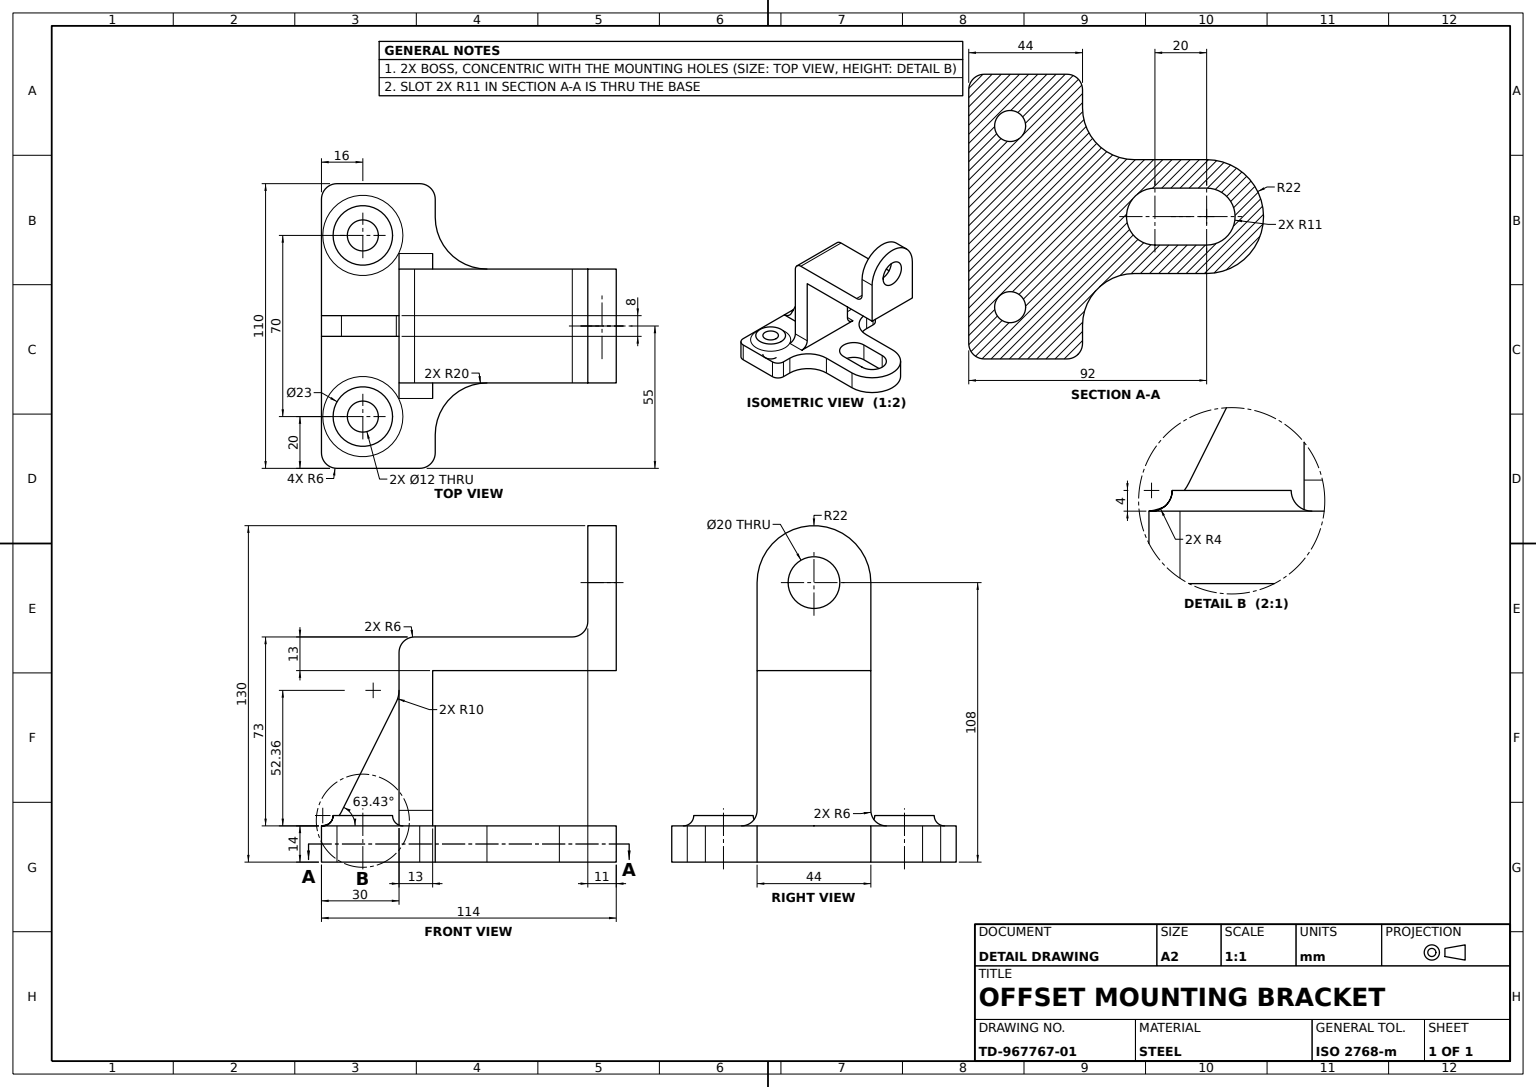
ISO-10303-21;
HEADER;
FILE_DESCRIPTION((''),'2;1');
FILE_NAME('','',(''),(''),'','','');
FILE_SCHEMA(('AUTOMOTIVE_DESIGN'));
ENDSEC;
DATA;
#1=APPLICATION_CONTEXT('');
#2=PRODUCT_CONTEXT('',#1,'mechanical');
#3=PRODUCT('','','',(#2));
#4=PRODUCT_DEFINITION_FORMATION('','',#3);
#5=PRODUCT_DEFINITION_CONTEXT('',#1,'design');
#6=PRODUCT_DEFINITION('','',#4,#5);
#7=PRODUCT_DEFINITION_SHAPE('','',#6);
#8=(LENGTH_UNIT()NAMED_UNIT(*)SI_UNIT(.MILLI.,.METRE.));
#9=(NAMED_UNIT(*)PLANE_ANGLE_UNIT()SI_UNIT($,.RADIAN.));
#10=(NAMED_UNIT(*)SI_UNIT($,.STERADIAN.)SOLID_ANGLE_UNIT());
#11=UNCERTAINTY_MEASURE_WITH_UNIT(LENGTH_MEASURE(1.E-05),#8,'distance_accuracy_value','');
#12=(GEOMETRIC_REPRESENTATION_CONTEXT(3)GLOBAL_UNCERTAINTY_ASSIGNED_CONTEXT((#11))GLOBAL_UNIT_ASSIGNED_CONTEXT((#8,#9,#10))REPRESENTATION_CONTEXT('',''));
#13=CARTESIAN_POINT('',(22.,20.,-43.));
#14=VERTEX_POINT('',#13);
#15=CARTESIAN_POINT('',(28.,14.,-43.));
#16=VERTEX_POINT('',#15);
#17=CARTESIAN_POINT('',(28.,20.,-43.));
#18=DIRECTION('',(0.,0.,1.));
#19=DIRECTION('',(0.,-1.,0.));
#20=AXIS2_PLACEMENT_3D('',#17,#18,#19);
#21=CIRCLE('',#20,6.);
#22=EDGE_CURVE('',#14,#16,#21,.T.);
#23=ORIENTED_EDGE('',*,*,#22,.T.);
#24=CARTESIAN_POINT('',(-28.,14.,-43.));
#25=VERTEX_POINT('',#24);
#26=CARTESIAN_POINT('',(22.,14.,-43.));
#27=DIRECTION('',(-1.,0.,0.));
#28=VECTOR('',#27,1000.);
#29=LINE('',#26,#28);
#30=EDGE_CURVE('',#16,#25,#29,.T.);
#31=ORIENTED_EDGE('',*,*,#30,.T.);
#32=CARTESIAN_POINT('',(-22.,20.,-43.));
#33=VERTEX_POINT('',#32);
#34=CARTESIAN_POINT('',(-28.,20.,-43.));
#35=AXIS2_PLACEMENT_3D('',#34,#18,#19);
#36=CIRCLE('',#35,6.);
#37=EDGE_CURVE('',#25,#33,#36,.T.);
#38=ORIENTED_EDGE('',*,*,#37,.T.);
#39=CARTESIAN_POINT('',(-22.,74.,-43.));
#40=VERTEX_POINT('',#39);
#41=DIRECTION('',(0.,1.,0.));
#42=VECTOR('',#41,1000.);
#43=LINE('',#39,#42);
#44=EDGE_CURVE('',#33,#40,#43,.T.);
#45=ORIENTED_EDGE('',*,*,#44,.T.);
#46=CARTESIAN_POINT('',(22.,74.,-43.));
#47=VERTEX_POINT('',#46);
#48=LINE('',#46,#28);
#49=EDGE_CURVE('',#47,#40,#48,.T.);
#50=ORIENTED_EDGE('',*,*,#49,.F.);
#51=LINE('',#46,#42);
#52=EDGE_CURVE('',#14,#47,#51,.T.);
#53=ORIENTED_EDGE('',*,*,#52,.F.);
#54=EDGE_LOOP('',(#23,#31,#38,#45,#50,#53));
#55=FACE_OUTER_BOUND('',#54,.T.);
#56=AXIS2_PLACEMENT_3D('',#46,#18,#19);
#57=PLANE('',#56);
#58=ADVANCED_FACE('',(#55),#57,.F.);
#59=CARTESIAN_POINT('',(-35.,18.,-4.5));
#60=VERTEX_POINT('',#59);
#61=CARTESIAN_POINT('',(-35.,18.,-27.5));
#62=VERTEX_POINT('',#61);
#63=CARTESIAN_POINT('',(-35.,18.,-16.));
#64=AXIS2_PLACEMENT_3D('',#63,#41,#18);
#65=CIRCLE('',#64,11.5);
#66=EDGE_CURVE('',#60,#62,#65,.T.);
#67=ORIENTED_EDGE('',*,*,#66,.T.);
#68=EDGE_CURVE('',#62,#60,#65,.T.);
#69=ORIENTED_EDGE('',*,*,#68,.T.);
#70=EDGE_LOOP('',(#67,#69));
#71=FACE_OUTER_BOUND('',#70,.T.);
#72=CARTESIAN_POINT('',(-35.,18.,-10.));
#73=VERTEX_POINT('',#72);
#74=CARTESIAN_POINT('',(-35.,18.,-22.));
#75=VERTEX_POINT('',#74);
#76=CIRCLE('',#64,6.);
#77=EDGE_CURVE('',#73,#75,#76,.T.);
#78=ORIENTED_EDGE('',*,*,#77,.F.);
#79=EDGE_CURVE('',#75,#73,#76,.T.);
#80=ORIENTED_EDGE('',*,*,#79,.F.);
#81=EDGE_LOOP('',(#78,#80));
#82=FACE_BOUND('',#81,.T.);
#83=PLANE('',#64);
#84=ADVANCED_FACE('',(#71,#82),#83,.T.);
#85=CARTESIAN_POINT('',(-35.,0.,-10.));
#86=VERTEX_POINT('',#85);
#87=CARTESIAN_POINT('',(-35.,0.,-22.));
#88=VERTEX_POINT('',#87);
#89=CARTESIAN_POINT('',(-35.,0.,-16.));
#90=AXIS2_PLACEMENT_3D('',#89,#41,#18);
#91=CIRCLE('',#90,6.);
#92=EDGE_CURVE('',#86,#88,#91,.T.);
#93=ORIENTED_EDGE('',*,*,#92,.F.);
#94=LINE('',#85,#42);
#95=EDGE_CURVE('',#86,#73,#94,.T.);
#96=ORIENTED_EDGE('',*,*,#95,.T.);
#97=ORIENTED_EDGE('',*,*,#77,.T.);
#98=LINE('',#87,#42);
#99=EDGE_CURVE('',#88,#75,#98,.T.);
#100=ORIENTED_EDGE('',*,*,#99,.F.);
#101=EDGE_LOOP('',(#93,#96,#97,#100));
#102=FACE_OUTER_BOUND('',#101,.T.);
#103=CYLINDRICAL_SURFACE('',#90,6.);
#104=ADVANCED_FACE('',(#102),#103,.F.);
#105=CARTESIAN_POINT('',(35.,18.,-27.5));
#106=VERTEX_POINT('',#105);
#107=CARTESIAN_POINT('',(35.,18.,-4.5));
#108=VERTEX_POINT('',#107);
#109=CARTESIAN_POINT('',(35.,18.,-16.));
#110=AXIS2_PLACEMENT_3D('',#109,#41,#18);
#111=CIRCLE('',#110,11.5);
#112=EDGE_CURVE('',#106,#108,#111,.T.);
#113=ORIENTED_EDGE('',*,*,#112,.T.);
#114=EDGE_CURVE('',#108,#106,#111,.T.);
#115=ORIENTED_EDGE('',*,*,#114,.T.);
#116=EDGE_LOOP('',(#113,#115));
#117=FACE_OUTER_BOUND('',#116,.T.);
#118=CARTESIAN_POINT('',(35.,18.,-10.));
#119=VERTEX_POINT('',#118);
#120=CARTESIAN_POINT('',(35.,18.,-22.));
#121=VERTEX_POINT('',#120);
#122=CIRCLE('',#110,6.);
#123=EDGE_CURVE('',#119,#121,#122,.T.);
#124=ORIENTED_EDGE('',*,*,#123,.F.);
#125=EDGE_CURVE('',#121,#119,#122,.T.);
#126=ORIENTED_EDGE('',*,*,#125,.F.);
#127=EDGE_LOOP('',(#124,#126));
#128=FACE_BOUND('',#127,.T.);
#129=PLANE('',#110);
#130=ADVANCED_FACE('',(#117,#128),#129,.T.);
#131=CARTESIAN_POINT('',(49.,0.,-44.));
#132=VERTEX_POINT('',#131);
#133=CARTESIAN_POINT('',(42.,0.,-44.));
#134=VERTEX_POINT('',#133);
#135=LINE('',#133,#28);
#136=EDGE_CURVE('',#132,#134,#135,.T.);
#137=ORIENTED_EDGE('',*,*,#136,.T.);
#138=CARTESIAN_POINT('',(42.,14.,-44.));
#139=VERTEX_POINT('',#138);
#140=VECTOR('',#19,1000.);
#141=LINE('',#138,#140);
#142=EDGE_CURVE('',#139,#134,#141,.T.);
#143=ORIENTED_EDGE('',*,*,#142,.F.);
#144=CARTESIAN_POINT('',(49.,14.,-44.));
#145=VERTEX_POINT('',#144);
#146=LINE('',#138,#28);
#147=EDGE_CURVE('',#145,#139,#146,.T.);
#148=ORIENTED_EDGE('',*,*,#147,.F.);
#149=LINE('',#144,#140);
#150=EDGE_CURVE('',#145,#132,#149,.T.);
#151=ORIENTED_EDGE('',*,*,#150,.T.);
#152=EDGE_LOOP('',(#137,#143,#148,#151));
#153=FACE_OUTER_BOUND('',#152,.T.);
#154=DIRECTION('',(1.,0.,0.));
#155=AXIS2_PLACEMENT_3D('',#138,#18,#154);
#156=PLANE('',#155);
#157=ADVANCED_FACE('',(#153),#156,.F.);
#158=CARTESIAN_POINT('',(22.,87.,-36.));
#159=VERTEX_POINT('',#158);
#160=CARTESIAN_POINT('',(-22.,87.,-36.));
#161=VERTEX_POINT('',#160);
#162=LINE('',#158,#28);
#163=EDGE_CURVE('',#159,#161,#162,.T.);
#164=ORIENTED_EDGE('',*,*,#163,.F.);
#165=CARTESIAN_POINT('',(22.,87.,-97.));
#166=VERTEX_POINT('',#165);
#167=VECTOR('',#18,1000.);
#168=LINE('',#158,#167);
#169=EDGE_CURVE('',#166,#159,#168,.T.);
#170=ORIENTED_EDGE('',*,*,#169,.F.);
#171=CARTESIAN_POINT('',(-22.,87.,-97.));
#172=VERTEX_POINT('',#171);
#173=LINE('',#171,#28);
#174=EDGE_CURVE('',#166,#172,#173,.T.);
#175=ORIENTED_EDGE('',*,*,#174,.T.);
#176=LINE('',#160,#167);
#177=EDGE_CURVE('',#172,#161,#176,.T.);
#178=ORIENTED_EDGE('',*,*,#177,.T.);
#179=EDGE_LOOP('',(#164,#170,#175,#178));
#180=FACE_OUTER_BOUND('',#179,.T.);
#181=DIRECTION('',(0.,0.,-1.));
#182=AXIS2_PLACEMENT_3D('',#158,#19,#181);
#183=PLANE('',#182);
#184=ADVANCED_FACE('',(#180),#183,.F.);
#185=CARTESIAN_POINT('',(-49.,14.,-44.));
#186=VERTEX_POINT('',#185);
#187=CARTESIAN_POINT('',(-49.,0.,-44.));
#188=VERTEX_POINT('',#187);
#189=LINE('',#185,#140);
#190=EDGE_CURVE('',#186,#188,#189,.T.);
#191=ORIENTED_EDGE('',*,*,#190,.T.);
#192=CARTESIAN_POINT('',(-55.,0.,-38.));
#193=VERTEX_POINT('',#192);
#194=CARTESIAN_POINT('',(-49.,0.,-38.));
#195=AXIS2_PLACEMENT_3D('',#194,#41,#18);
#196=CIRCLE('',#195,6.);
#197=EDGE_CURVE('',#188,#193,#196,.T.);
#198=ORIENTED_EDGE('',*,*,#197,.T.);
#199=CARTESIAN_POINT('',(-55.,14.,-38.));
#200=VERTEX_POINT('',#199);
#201=LINE('',#199,#140);
#202=EDGE_CURVE('',#200,#193,#201,.T.);
#203=ORIENTED_EDGE('',*,*,#202,.F.);
#204=CARTESIAN_POINT('',(-49.,14.,-38.));
#205=AXIS2_PLACEMENT_3D('',#204,#41,#18);
#206=CIRCLE('',#205,6.);
#207=EDGE_CURVE('',#186,#200,#206,.T.);
#208=ORIENTED_EDGE('',*,*,#207,.F.);
#209=EDGE_LOOP('',(#191,#198,#203,#208));
#210=FACE_OUTER_BOUND('',#209,.T.);
#211=AXIS2_PLACEMENT_3D('',#204,#19,#181);
#212=CYLINDRICAL_SURFACE('',#211,6.);
#213=ADVANCED_FACE('',(#210),#212,.T.);
#214=CARTESIAN_POINT('',(55.,14.,-6.));
#215=VERTEX_POINT('',#214);
#216=CARTESIAN_POINT('',(55.,0.,-6.));
#217=VERTEX_POINT('',#216);
#218=LINE('',#214,#140);
#219=EDGE_CURVE('',#215,#217,#218,.T.);
#220=ORIENTED_EDGE('',*,*,#219,.T.);
#221=CARTESIAN_POINT('',(55.,0.,-38.));
#222=VERTEX_POINT('',#221);
#223=VECTOR('',#181,1000.);
#224=LINE('',#216,#223);
#225=EDGE_CURVE('',#217,#222,#224,.T.);
#226=ORIENTED_EDGE('',*,*,#225,.T.);
#227=CARTESIAN_POINT('',(55.,14.,-38.));
#228=VERTEX_POINT('',#227);
#229=LINE('',#227,#140);
#230=EDGE_CURVE('',#228,#222,#229,.T.);
#231=ORIENTED_EDGE('',*,*,#230,.F.);
#232=LINE('',#214,#223);
#233=EDGE_CURVE('',#215,#228,#232,.T.);
#234=ORIENTED_EDGE('',*,*,#233,.F.);
#235=EDGE_LOOP('',(#220,#226,#231,#234));
#236=FACE_OUTER_BOUND('',#235,.T.);
#237=AXIS2_PLACEMENT_3D('',#214,#27,#18);
#238=PLANE('',#237);
#239=ADVANCED_FACE('',(#236),#238,.F.);
#240=CARTESIAN_POINT('',(0.,14.,-103.));
#241=VERTEX_POINT('',#240);
#242=CARTESIAN_POINT('',(-11.,14.,-92.));
#243=VERTEX_POINT('',#242);
#244=CARTESIAN_POINT('',(0.,14.,-92.));
#245=AXIS2_PLACEMENT_3D('',#244,#41,#18);
#246=CIRCLE('',#245,11.);
#247=EDGE_CURVE('',#241,#243,#246,.T.);
#248=ORIENTED_EDGE('',*,*,#247,.T.);
#249=CARTESIAN_POINT('',(-11.,0.,-92.));
#250=VERTEX_POINT('',#249);
#251=LINE('',#242,#140);
#252=EDGE_CURVE('',#243,#250,#251,.T.);
#253=ORIENTED_EDGE('',*,*,#252,.T.);
#254=CARTESIAN_POINT('',(0.,0.,-103.));
#255=VERTEX_POINT('',#254);
#256=CARTESIAN_POINT('',(0.,0.,-92.));
#257=AXIS2_PLACEMENT_3D('',#256,#41,#18);
#258=CIRCLE('',#257,11.);
#259=EDGE_CURVE('',#255,#250,#258,.T.);
#260=ORIENTED_EDGE('',*,*,#259,.F.);
#261=LINE('',#240,#140);
#262=EDGE_CURVE('',#241,#255,#261,.T.);
#263=ORIENTED_EDGE('',*,*,#262,.F.);
#264=EDGE_LOOP('',(#248,#253,#260,#263));
#265=FACE_OUTER_BOUND('',#264,.T.);
#266=AXIS2_PLACEMENT_3D('',#244,#19,#181);
#267=CYLINDRICAL_SURFACE('',#266,11.);
#268=ADVANCED_FACE('',(#265),#267,.F.);
#269=CARTESIAN_POINT('',(-4.,19.453467,-7.726734));
#270=VERTEX_POINT('',#269);
#271=CARTESIAN_POINT('',(-4.,61.888544,-28.944272));
#272=VERTEX_POINT('',#271);
#273=CARTESIAN_POINT('',(-4.,14.,-5.));
#274=DIRECTION('',(0.,0.894427191,-0.447213595));
#275=VECTOR('',#274,1000.);
#276=LINE('',#273,#275);
#277=EDGE_CURVE('',#270,#272,#276,.T.);
#278=ORIENTED_EDGE('',*,*,#277,.F.);
#279=CARTESIAN_POINT('',(4.,19.453467,-7.726734));
#280=VERTEX_POINT('',#279);
#281=VECTOR('',#154,1000.);
#282=LINE('',#279,#281);
#283=EDGE_CURVE('',#270,#280,#282,.T.);
#284=ORIENTED_EDGE('',*,*,#283,.T.);
#285=CARTESIAN_POINT('',(4.,61.888544,-28.944272));
#286=VERTEX_POINT('',#285);
#287=CARTESIAN_POINT('',(4.,14.,-5.));
#288=LINE('',#287,#275);
#289=EDGE_CURVE('',#280,#286,#288,.T.);
#290=ORIENTED_EDGE('',*,*,#289,.T.);
#291=CARTESIAN_POINT('',(0.,61.888544,-28.944272));
#292=LINE('',#291,#28);
#293=EDGE_CURVE('',#286,#272,#292,.T.);
#294=ORIENTED_EDGE('',*,*,#293,.T.);
#295=EDGE_LOOP('',(#278,#284,#290,#294));
#296=FACE_OUTER_BOUND('',#295,.T.);
#297=CARTESIAN_POINT('',(0.,14.,-5.));
#298=DIRECTION('',(0.,-0.447213595,-0.894427191));
#299=AXIS2_PLACEMENT_3D('',#297,#298,#274);
#300=PLANE('',#299);
#301=ADVANCED_FACE('',(#296),#300,.F.);
#302=CARTESIAN_POINT('',(-22.,14.,-64.));
#303=VERTEX_POINT('',#302);
#304=CARTESIAN_POINT('',(-42.,14.,-44.));
#305=VERTEX_POINT('',#304);
#306=CARTESIAN_POINT('',(-42.,14.,-64.));
#307=AXIS2_PLACEMENT_3D('',#306,#19,#18);
#308=CIRCLE('',#307,20.);
#309=EDGE_CURVE('',#303,#305,#308,.T.);
#310=ORIENTED_EDGE('',*,*,#309,.F.);
#311=CARTESIAN_POINT('',(-22.,0.,-64.));
#312=VERTEX_POINT('',#311);
#313=LINE('',#302,#140);
#314=EDGE_CURVE('',#303,#312,#313,.T.);
#315=ORIENTED_EDGE('',*,*,#314,.T.);
#316=CARTESIAN_POINT('',(-42.,0.,-44.));
#317=VERTEX_POINT('',#316);
#318=CARTESIAN_POINT('',(-42.,0.,-64.));
#319=AXIS2_PLACEMENT_3D('',#318,#19,#18);
#320=CIRCLE('',#319,20.);
#321=EDGE_CURVE('',#312,#317,#320,.T.);
#322=ORIENTED_EDGE('',*,*,#321,.T.);
#323=LINE('',#304,#140);
#324=EDGE_CURVE('',#305,#317,#323,.T.);
#325=ORIENTED_EDGE('',*,*,#324,.F.);
#326=EDGE_LOOP('',(#310,#315,#322,#325));
#327=FACE_OUTER_BOUND('',#326,.T.);
#328=AXIS2_PLACEMENT_3D('',#306,#19,#181);
#329=CYLINDRICAL_SURFACE('',#328,20.);
#330=ADVANCED_FACE('',(#327),#329,.F.);
#331=CARTESIAN_POINT('',(-11.,0.,-72.));
#332=VERTEX_POINT('',#331);
#333=CARTESIAN_POINT('',(11.,0.,-72.));
#334=VERTEX_POINT('',#333);
#335=CARTESIAN_POINT('',(0.,0.,-72.));
#336=AXIS2_PLACEMENT_3D('',#335,#41,#18);
#337=CIRCLE('',#336,11.);
#338=EDGE_CURVE('',#332,#334,#337,.T.);
#339=ORIENTED_EDGE('',*,*,#338,.F.);
#340=CARTESIAN_POINT('',(-11.,14.,-72.));
#341=VERTEX_POINT('',#340);
#342=LINE('',#340,#140);
#343=EDGE_CURVE('',#341,#332,#342,.T.);
#344=ORIENTED_EDGE('',*,*,#343,.F.);
#345=CARTESIAN_POINT('',(11.,14.,-72.));
#346=VERTEX_POINT('',#345);
#347=CARTESIAN_POINT('',(0.,14.,-72.));
#348=AXIS2_PLACEMENT_3D('',#347,#41,#18);
#349=CIRCLE('',#348,11.);
#350=EDGE_CURVE('',#341,#346,#349,.T.);
#351=ORIENTED_EDGE('',*,*,#350,.T.);
#352=LINE('',#345,#140);
#353=EDGE_CURVE('',#346,#334,#352,.T.);
#354=ORIENTED_EDGE('',*,*,#353,.T.);
#355=EDGE_LOOP('',(#339,#344,#351,#354));
#356=FACE_OUTER_BOUND('',#355,.T.);
#357=AXIS2_PLACEMENT_3D('',#347,#19,#181);
#358=CYLINDRICAL_SURFACE('',#357,11.);
#359=ADVANCED_FACE('',(#356),#358,.F.);
#360=CARTESIAN_POINT('',(-22.,14.,-92.));
#361=VERTEX_POINT('',#360);
#362=LINE('',#302,#167);
#363=EDGE_CURVE('',#361,#303,#362,.T.);
#364=ORIENTED_EDGE('',*,*,#363,.F.);
#365=CARTESIAN_POINT('',(-22.,0.,-92.));
#366=VERTEX_POINT('',#365);
#367=LINE('',#360,#140);
#368=EDGE_CURVE('',#361,#366,#367,.T.);
#369=ORIENTED_EDGE('',*,*,#368,.T.);
#370=LINE('',#311,#167);
#371=EDGE_CURVE('',#366,#312,#370,.T.);
#372=ORIENTED_EDGE('',*,*,#371,.T.);
#373=ORIENTED_EDGE('',*,*,#314,.F.);
#374=EDGE_LOOP('',(#364,#369,#372,#373));
#375=FACE_OUTER_BOUND('',#374,.T.);
#376=AXIS2_PLACEMENT_3D('',#302,#154,#181);
#377=PLANE('',#376);
#378=ADVANCED_FACE('',(#375),#377,.F.);
#379=CARTESIAN_POINT('',(-22.,74.,-114.));
#380=VERTEX_POINT('',#379);
#381=LINE('',#379,#223);
#382=EDGE_CURVE('',#40,#380,#381,.T.);
#383=ORIENTED_EDGE('',*,*,#382,.F.);
#384=ORIENTED_EDGE('',*,*,#44,.F.);
#385=CARTESIAN_POINT('',(-22.,20.,-30.));
#386=VERTEX_POINT('',#385);
#387=LINE('',#385,#167);
#388=EDGE_CURVE('',#33,#386,#387,.T.);
#389=ORIENTED_EDGE('',*,*,#388,.T.);
#390=CARTESIAN_POINT('',(-22.,81.,-30.));
#391=VERTEX_POINT('',#390);
#392=CARTESIAN_POINT('',(-22.,14.,-30.));
#393=LINE('',#392,#140);
#394=EDGE_CURVE('',#391,#386,#393,.T.);
#395=ORIENTED_EDGE('',*,*,#394,.F.);
#396=CARTESIAN_POINT('',(-22.,81.,-36.));
#397=AXIS2_PLACEMENT_3D('',#396,#154,#18);
#398=CIRCLE('',#397,6.);
#399=EDGE_CURVE('',#161,#391,#398,.T.);
#400=ORIENTED_EDGE('',*,*,#399,.F.);
#401=ORIENTED_EDGE('',*,*,#177,.F.);
#402=CARTESIAN_POINT('',(-22.,93.,-103.));
#403=VERTEX_POINT('',#402);
#404=CARTESIAN_POINT('',(-22.,93.,-97.));
#405=AXIS2_PLACEMENT_3D('',#404,#154,#18);
#406=CIRCLE('',#405,6.);
#407=EDGE_CURVE('',#172,#403,#406,.T.);
#408=ORIENTED_EDGE('',*,*,#407,.T.);
#409=CARTESIAN_POINT('',(-22.,108.,-103.));
#410=VERTEX_POINT('',#409);
#411=CARTESIAN_POINT('',(-22.,87.,-103.));
#412=LINE('',#411,#140);
#413=EDGE_CURVE('',#410,#403,#412,.T.);
#414=ORIENTED_EDGE('',*,*,#413,.F.);
#415=CARTESIAN_POINT('',(-22.,108.,-114.));
#416=VERTEX_POINT('',#415);
#417=LINE('',#409,#167);
#418=EDGE_CURVE('',#416,#410,#417,.T.);
#419=ORIENTED_EDGE('',*,*,#418,.F.);
#420=LINE('',#415,#42);
#421=EDGE_CURVE('',#380,#416,#420,.T.);
#422=ORIENTED_EDGE('',*,*,#421,.F.);
#423=EDGE_LOOP('',(#383,#384,#389,#395,#400,#401,#408,#414,#419,#422));
#424=FACE_OUTER_BOUND('',#423,.T.);
#425=AXIS2_PLACEMENT_3D('',#396,#27,#18);
#426=PLANE('',#425);
#427=ADVANCED_FACE('',(#424),#426,.T.);
#428=CARTESIAN_POINT('',(35.,14.,-31.5));
#429=VERTEX_POINT('',#428);
#430=CARTESIAN_POINT('',(35.,14.,-0.5));
#431=VERTEX_POINT('',#430);
#432=CARTESIAN_POINT('',(35.,14.,-16.));
#433=AXIS2_PLACEMENT_3D('',#432,#19,#18);
#434=CIRCLE('',#433,15.5);
#435=EDGE_CURVE('',#429,#431,#434,.T.);
#436=ORIENTED_EDGE('',*,*,#435,.F.);
#437=CARTESIAN_POINT('',(35.,18.,-31.5));
#438=AXIS2_PLACEMENT_3D('',#437,#154,#181);
#439=CIRCLE('',#438,4.);
#440=EDGE_CURVE('',#106,#429,#439,.T.);
#441=ORIENTED_EDGE('',*,*,#440,.F.);
#442=ORIENTED_EDGE('',*,*,#114,.F.);
#443=CARTESIAN_POINT('',(35.,18.,-0.5));
#444=AXIS2_PLACEMENT_3D('',#443,#27,#18);
#445=CIRCLE('',#444,4.);
#446=EDGE_CURVE('',#108,#431,#445,.T.);
#447=ORIENTED_EDGE('',*,*,#446,.T.);
#448=EDGE_LOOP('',(#436,#441,#442,#447));
#449=FACE_OUTER_BOUND('',#448,.T.);
#450=TOROIDAL_SURFACE('',#110,15.5,4.);
#451=ADVANCED_FACE('',(#449),#450,.F.);
#452=CARTESIAN_POINT('',(10.,108.,-103.));
#453=VERTEX_POINT('',#452);
#454=CARTESIAN_POINT('',(10.,108.,-114.));
#455=VERTEX_POINT('',#454);
#456=CARTESIAN_POINT('',(10.,108.,0.001));
#457=LINE('',#456,#223);
#458=EDGE_CURVE('',#453,#455,#457,.T.);
#459=ORIENTED_EDGE('',*,*,#458,.F.);
#460=CARTESIAN_POINT('',(-10.,108.,-103.));
#461=VERTEX_POINT('',#460);
#462=CARTESIAN_POINT('',(0.,108.,-103.));
#463=AXIS2_PLACEMENT_3D('',#462,#18,#41);
#464=CIRCLE('',#463,10.);
#465=EDGE_CURVE('',#453,#461,#464,.T.);
#466=ORIENTED_EDGE('',*,*,#465,.T.);
#467=CARTESIAN_POINT('',(-10.,108.,-114.));
#468=VERTEX_POINT('',#467);
#469=CARTESIAN_POINT('',(-10.,108.,0.001));
#470=LINE('',#469,#223);
#471=EDGE_CURVE('',#461,#468,#470,.T.);
#472=ORIENTED_EDGE('',*,*,#471,.T.);
#473=CARTESIAN_POINT('',(0.,108.,-114.));
#474=AXIS2_PLACEMENT_3D('',#473,#181,#27);
#475=CIRCLE('',#474,10.);
#476=EDGE_CURVE('',#468,#455,#475,.T.);
#477=ORIENTED_EDGE('',*,*,#476,.T.);
#478=EDGE_LOOP('',(#459,#466,#472,#477));
#479=FACE_OUTER_BOUND('',#478,.T.);
#480=CARTESIAN_POINT('',(0.,108.,0.001));
#481=AXIS2_PLACEMENT_3D('',#480,#181,#27);
#482=CYLINDRICAL_SURFACE('',#481,10.);
#483=ADVANCED_FACE('',(#479),#482,.F.);
#484=CARTESIAN_POINT('',(22.,93.,-103.));
#485=VERTEX_POINT('',#484);
#486=LINE('',#484,#281);
#487=EDGE_CURVE('',#403,#485,#486,.T.);
#488=ORIENTED_EDGE('',*,*,#487,.T.);
#489=CARTESIAN_POINT('',(22.,108.,-103.));
#490=VERTEX_POINT('',#489);
#491=CARTESIAN_POINT('',(22.,87.,-103.));
#492=LINE('',#491,#140);
#493=EDGE_CURVE('',#490,#485,#492,.T.);
#494=ORIENTED_EDGE('',*,*,#493,.F.);
#495=CIRCLE('',#463,22.);
#496=EDGE_CURVE('',#490,#410,#495,.T.);
#497=ORIENTED_EDGE('',*,*,#496,.T.);
#498=ORIENTED_EDGE('',*,*,#413,.T.);
#499=EDGE_LOOP('',(#488,#494,#497,#498));
#500=FACE_OUTER_BOUND('',#499,.T.);
#501=EDGE_CURVE('',#461,#453,#464,.T.);
#502=ORIENTED_EDGE('',*,*,#501,.F.);
#503=ORIENTED_EDGE('',*,*,#465,.F.);
#504=EDGE_LOOP('',(#502,#503));
#505=FACE_BOUND('',#504,.T.);
#506=AXIS2_PLACEMENT_3D('',#491,#181,#41);
#507=PLANE('',#506);
#508=ADVANCED_FACE('',(#500,#505),#507,.F.);
#509=CARTESIAN_POINT('',(49.,14.,-38.));
#510=AXIS2_PLACEMENT_3D('',#509,#41,#18);
#511=CIRCLE('',#510,6.);
#512=EDGE_CURVE('',#228,#145,#511,.T.);
#513=ORIENTED_EDGE('',*,*,#512,.T.);
#514=ORIENTED_EDGE('',*,*,#147,.T.);
#515=CARTESIAN_POINT('',(22.,14.,-64.));
#516=VERTEX_POINT('',#515);
#517=CARTESIAN_POINT('',(42.,14.,-64.));
#518=AXIS2_PLACEMENT_3D('',#517,#19,#18);
#519=CIRCLE('',#518,20.);
#520=EDGE_CURVE('',#139,#516,#519,.T.);
#521=ORIENTED_EDGE('',*,*,#520,.T.);
#522=CARTESIAN_POINT('',(22.,14.,-92.));
#523=VERTEX_POINT('',#522);
#524=LINE('',#522,#223);
#525=EDGE_CURVE('',#516,#523,#524,.T.);
#526=ORIENTED_EDGE('',*,*,#525,.T.);
#527=CARTESIAN_POINT('',(0.,14.,-114.));
#528=VERTEX_POINT('',#527);
#529=AXIS2_PLACEMENT_3D('',#244,#41,#181);
#530=CIRCLE('',#529,22.);
#531=EDGE_CURVE('',#523,#528,#530,.T.);
#532=ORIENTED_EDGE('',*,*,#531,.T.);
#533=EDGE_CURVE('',#528,#361,#530,.T.);
#534=ORIENTED_EDGE('',*,*,#533,.T.);
#535=ORIENTED_EDGE('',*,*,#363,.T.);
#536=ORIENTED_EDGE('',*,*,#309,.T.);
#537=LINE('',#185,#28);
#538=EDGE_CURVE('',#305,#186,#537,.T.);
#539=ORIENTED_EDGE('',*,*,#538,.T.);
#540=ORIENTED_EDGE('',*,*,#207,.T.);
#541=CARTESIAN_POINT('',(-55.,14.,-6.));
#542=VERTEX_POINT('',#541);
#543=LINE('',#199,#167);
#544=EDGE_CURVE('',#200,#542,#543,.T.);
#545=ORIENTED_EDGE('',*,*,#544,.T.);
#546=CARTESIAN_POINT('',(-49.,14.,0.));
#547=VERTEX_POINT('',#546);
#548=CARTESIAN_POINT('',(-49.,14.,-6.));
#549=AXIS2_PLACEMENT_3D('',#548,#41,#18);
#550=CIRCLE('',#549,6.);
#551=EDGE_CURVE('',#542,#547,#550,.T.);
#552=ORIENTED_EDGE('',*,*,#551,.T.);
#553=CARTESIAN_POINT('',(-4.,14.,0.));
#554=VERTEX_POINT('',#553);
#555=LINE('',#546,#281);
#556=EDGE_CURVE('',#547,#554,#555,.T.);
#557=ORIENTED_EDGE('',*,*,#556,.T.);
#558=CARTESIAN_POINT('',(-4.,14.,-30.));
#559=VERTEX_POINT('',#558);
#560=CARTESIAN_POINT('',(-4.,14.,-6.));
#561=LINE('',#560,#223);
#562=EDGE_CURVE('',#554,#559,#561,.T.);
#563=ORIENTED_EDGE('',*,*,#562,.T.);
#564=CARTESIAN_POINT('',(-28.,14.,-30.));
#565=VERTEX_POINT('',#564);
#566=CARTESIAN_POINT('',(22.,14.,-30.));
#567=LINE('',#566,#28);
#568=EDGE_CURVE('',#559,#565,#567,.T.);
#569=ORIENTED_EDGE('',*,*,#568,.T.);
#570=LINE('',#24,#223);
#571=EDGE_CURVE('',#565,#25,#570,.T.);
#572=ORIENTED_EDGE('',*,*,#571,.T.);
#573=ORIENTED_EDGE('',*,*,#30,.F.);
#574=CARTESIAN_POINT('',(28.,14.,-30.));
#575=VERTEX_POINT('',#574);
#576=CARTESIAN_POINT('',(28.,14.,-6.));
#577=LINE('',#576,#167);
#578=EDGE_CURVE('',#16,#575,#577,.T.);
#579=ORIENTED_EDGE('',*,*,#578,.T.);
#580=CARTESIAN_POINT('',(4.,14.,-30.));
#581=VERTEX_POINT('',#580);
#582=EDGE_CURVE('',#575,#581,#567,.T.);
#583=ORIENTED_EDGE('',*,*,#582,.T.);
#584=CARTESIAN_POINT('',(4.,14.,0.));
#585=VERTEX_POINT('',#584);
#586=CARTESIAN_POINT('',(4.,14.,-6.));
#587=LINE('',#586,#223);
#588=EDGE_CURVE('',#585,#581,#587,.T.);
#589=ORIENTED_EDGE('',*,*,#588,.F.);
#590=CARTESIAN_POINT('',(49.,14.,0.));
#591=VERTEX_POINT('',#590);
#592=EDGE_CURVE('',#585,#591,#555,.T.);
#593=ORIENTED_EDGE('',*,*,#592,.T.);
#594=CARTESIAN_POINT('',(49.,14.,-6.));
#595=AXIS2_PLACEMENT_3D('',#594,#41,#18);
#596=CIRCLE('',#595,6.);
#597=EDGE_CURVE('',#591,#215,#596,.T.);
#598=ORIENTED_EDGE('',*,*,#597,.T.);
#599=ORIENTED_EDGE('',*,*,#233,.T.);
#600=EDGE_LOOP('',(#513,#514,#521,#526,#532,#534,#535,#536,#539,#540,#545,#552,#557,#563,#569,#572,#573,#579,#583,#589,#593,#598,#599));
#601=FACE_OUTER_BOUND('',#600,.T.);
#602=ORIENTED_EDGE('',*,*,#435,.T.);
#603=EDGE_CURVE('',#431,#429,#434,.T.);
#604=ORIENTED_EDGE('',*,*,#603,.T.);
#605=EDGE_LOOP('',(#602,#604));
#606=FACE_BOUND('',#605,.T.);
#607=CARTESIAN_POINT('',(-35.,14.,-0.5));
#608=VERTEX_POINT('',#607);
#609=CARTESIAN_POINT('',(-35.,14.,-31.5));
#610=VERTEX_POINT('',#609);
#611=CARTESIAN_POINT('',(-35.,14.,-16.));
#612=AXIS2_PLACEMENT_3D('',#611,#19,#18);
#613=CIRCLE('',#612,15.5);
#614=EDGE_CURVE('',#608,#610,#613,.T.);
#615=ORIENTED_EDGE('',*,*,#614,.T.);
#616=EDGE_CURVE('',#610,#608,#613,.T.);
#617=ORIENTED_EDGE('',*,*,#616,.T.);
#618=EDGE_LOOP('',(#615,#617));
#619=FACE_BOUND('',#618,.T.);
#620=CARTESIAN_POINT('',(11.,14.,-92.));
#621=VERTEX_POINT('',#620);
#622=LINE('',#620,#223);
#623=EDGE_CURVE('',#346,#621,#622,.T.);
#624=ORIENTED_EDGE('',*,*,#623,.F.);
#625=ORIENTED_EDGE('',*,*,#350,.F.);
#626=LINE('',#242,#167);
#627=EDGE_CURVE('',#243,#341,#626,.T.);
#628=ORIENTED_EDGE('',*,*,#627,.F.);
#629=ORIENTED_EDGE('',*,*,#247,.F.);
#630=EDGE_CURVE('',#621,#241,#246,.T.);
#631=ORIENTED_EDGE('',*,*,#630,.F.);
#632=EDGE_LOOP('',(#624,#625,#628,#629,#631));
#633=FACE_BOUND('',#632,.T.);
#634=PLANE('',#595);
#635=ADVANCED_FACE('',(#601,#606,#619,#633),#634,.T.);
#636=CARTESIAN_POINT('',(-35.,18.,-31.5));
#637=AXIS2_PLACEMENT_3D('',#636,#154,#181);
#638=CIRCLE('',#637,4.);
#639=EDGE_CURVE('',#62,#610,#638,.T.);
#640=ORIENTED_EDGE('',*,*,#639,.F.);
#641=ORIENTED_EDGE('',*,*,#66,.F.);
#642=CARTESIAN_POINT('',(-35.,18.,-0.5));
#643=AXIS2_PLACEMENT_3D('',#642,#27,#18);
#644=CIRCLE('',#643,4.);
#645=EDGE_CURVE('',#60,#608,#644,.T.);
#646=ORIENTED_EDGE('',*,*,#645,.T.);
#647=ORIENTED_EDGE('',*,*,#616,.F.);
#648=EDGE_LOOP('',(#640,#641,#646,#647));
#649=FACE_OUTER_BOUND('',#648,.T.);
#650=TOROIDAL_SURFACE('',#64,15.5,4.);
#651=ADVANCED_FACE('',(#649),#650,.F.);
#652=ORIENTED_EDGE('',*,*,#525,.F.);
#653=CARTESIAN_POINT('',(22.,0.,-64.));
#654=VERTEX_POINT('',#653);
#655=LINE('',#515,#140);
#656=EDGE_CURVE('',#516,#654,#655,.T.);
#657=ORIENTED_EDGE('',*,*,#656,.T.);
#658=CARTESIAN_POINT('',(22.,0.,-92.));
#659=VERTEX_POINT('',#658);
#660=LINE('',#658,#223);
#661=EDGE_CURVE('',#654,#659,#660,.T.);
#662=ORIENTED_EDGE('',*,*,#661,.T.);
#663=LINE('',#522,#140);
#664=EDGE_CURVE('',#523,#659,#663,.T.);
#665=ORIENTED_EDGE('',*,*,#664,.F.);
#666=EDGE_LOOP('',(#652,#657,#662,#665));
#667=FACE_OUTER_BOUND('',#666,.T.);
#668=AXIS2_PLACEMENT_3D('',#522,#27,#18);
#669=PLANE('',#668);
#670=ADVANCED_FACE('',(#667),#669,.F.);
#671=CARTESIAN_POINT('',(22.,108.,-114.));
#672=VERTEX_POINT('',#671);
#673=CIRCLE('',#474,22.);
#674=EDGE_CURVE('',#416,#672,#673,.T.);
#675=ORIENTED_EDGE('',*,*,#674,.F.);
#676=ORIENTED_EDGE('',*,*,#418,.T.);
#677=ORIENTED_EDGE('',*,*,#496,.F.);
#678=LINE('',#489,#167);
#679=EDGE_CURVE('',#672,#490,#678,.T.);
#680=ORIENTED_EDGE('',*,*,#679,.F.);
#681=EDGE_LOOP('',(#675,#676,#677,#680));
#682=FACE_OUTER_BOUND('',#681,.T.);
#683=CARTESIAN_POINT('',(0.,108.,-40.774603));
#684=AXIS2_PLACEMENT_3D('',#683,#181,#27);
#685=CYLINDRICAL_SURFACE('',#684,22.);
#686=ADVANCED_FACE('',(#682),#685,.T.);
#687=CARTESIAN_POINT('',(-4.,66.36068,-30.));
#688=VERTEX_POINT('',#687);
#689=CARTESIAN_POINT('',(4.,66.36068,-30.));
#690=VERTEX_POINT('',#689);
#691=CARTESIAN_POINT('',(22.,66.36068,-30.));
#692=LINE('',#691,#281);
#693=EDGE_CURVE('',#688,#690,#692,.T.);
#694=ORIENTED_EDGE('',*,*,#693,.F.);
#695=CARTESIAN_POINT('',(-4.,66.36068,-20.));
#696=AXIS2_PLACEMENT_3D('',#695,#154,#181);
#697=CIRCLE('',#696,10.);
#698=EDGE_CURVE('',#272,#688,#697,.T.);
#699=ORIENTED_EDGE('',*,*,#698,.F.);
#700=ORIENTED_EDGE('',*,*,#293,.F.);
#701=CARTESIAN_POINT('',(4.,66.36068,-20.));
#702=AXIS2_PLACEMENT_3D('',#701,#27,#181);
#703=CIRCLE('',#702,10.);
#704=EDGE_CURVE('',#690,#286,#703,.T.);
#705=ORIENTED_EDGE('',*,*,#704,.F.);
#706=EDGE_LOOP('',(#694,#699,#700,#705));
#707=FACE_OUTER_BOUND('',#706,.T.);
#708=CARTESIAN_POINT('',(22.,66.36068,-20.));
#709=AXIS2_PLACEMENT_3D('',#708,#27,#18);
#710=CYLINDRICAL_SURFACE('',#709,10.);
#711=ADVANCED_FACE('',(#707),#710,.F.);
#712=EDGE_CURVE('',#455,#468,#475,.T.);
#713=ORIENTED_EDGE('',*,*,#712,.F.);
#714=ORIENTED_EDGE('',*,*,#476,.F.);
#715=EDGE_LOOP('',(#713,#714));
#716=FACE_BOUND('',#715,.T.);
#717=ORIENTED_EDGE('',*,*,#674,.T.);
#718=CARTESIAN_POINT('',(22.,74.,-114.));
#719=VERTEX_POINT('',#718);
#720=LINE('',#671,#42);
#721=EDGE_CURVE('',#719,#672,#720,.T.);
#722=ORIENTED_EDGE('',*,*,#721,.F.);
#723=LINE('',#718,#28);
#724=EDGE_CURVE('',#719,#380,#723,.T.);
#725=ORIENTED_EDGE('',*,*,#724,.T.);
#726=ORIENTED_EDGE('',*,*,#421,.T.);
#727=EDGE_LOOP('',(#717,#722,#725,#726));
#728=FACE_OUTER_BOUND('',#727,.T.);
#729=AXIS2_PLACEMENT_3D('',#671,#18,#154);
#730=PLANE('',#729);
#731=ADVANCED_FACE('',(#716,#728),#730,.F.);
#732=ORIENTED_EDGE('',*,*,#321,.F.);
#733=ORIENTED_EDGE('',*,*,#371,.F.);
#734=CARTESIAN_POINT('',(0.,0.,-114.));
#735=VERTEX_POINT('',#734);
#736=AXIS2_PLACEMENT_3D('',#256,#41,#181);
#737=CIRCLE('',#736,22.);
#738=EDGE_CURVE('',#735,#366,#737,.T.);
#739=ORIENTED_EDGE('',*,*,#738,.F.);
#740=EDGE_CURVE('',#659,#735,#737,.T.);
#741=ORIENTED_EDGE('',*,*,#740,.F.);
#742=ORIENTED_EDGE('',*,*,#661,.F.);
#743=CARTESIAN_POINT('',(42.,0.,-64.));
#744=AXIS2_PLACEMENT_3D('',#743,#19,#18);
#745=CIRCLE('',#744,20.);
#746=EDGE_CURVE('',#134,#654,#745,.T.);
#747=ORIENTED_EDGE('',*,*,#746,.F.);
#748=ORIENTED_EDGE('',*,*,#136,.F.);
#749=CARTESIAN_POINT('',(49.,0.,-38.));
#750=AXIS2_PLACEMENT_3D('',#749,#41,#18);
#751=CIRCLE('',#750,6.);
#752=EDGE_CURVE('',#222,#132,#751,.T.);
#753=ORIENTED_EDGE('',*,*,#752,.F.);
#754=ORIENTED_EDGE('',*,*,#225,.F.);
#755=CARTESIAN_POINT('',(49.,0.,0.));
#756=VERTEX_POINT('',#755);
#757=CARTESIAN_POINT('',(49.,0.,-6.));
#758=AXIS2_PLACEMENT_3D('',#757,#41,#18);
#759=CIRCLE('',#758,6.);
#760=EDGE_CURVE('',#756,#217,#759,.T.);
#761=ORIENTED_EDGE('',*,*,#760,.F.);
#762=CARTESIAN_POINT('',(-49.,0.,0.));
#763=VERTEX_POINT('',#762);
#764=CARTESIAN_POINT('',(0.,0.,0.));
#765=LINE('',#764,#281);
#766=EDGE_CURVE('',#763,#756,#765,.T.);
#767=ORIENTED_EDGE('',*,*,#766,.F.);
#768=CARTESIAN_POINT('',(-55.,0.,-6.));
#769=VERTEX_POINT('',#768);
#770=CARTESIAN_POINT('',(-49.,0.,-6.));
#771=AXIS2_PLACEMENT_3D('',#770,#41,#18);
#772=CIRCLE('',#771,6.);
#773=EDGE_CURVE('',#769,#763,#772,.T.);
#774=ORIENTED_EDGE('',*,*,#773,.F.);
#775=LINE('',#192,#167);
#776=EDGE_CURVE('',#193,#769,#775,.T.);
#777=ORIENTED_EDGE('',*,*,#776,.F.);
#778=ORIENTED_EDGE('',*,*,#197,.F.);
#779=LINE('',#187,#28);
#780=EDGE_CURVE('',#317,#188,#779,.T.);
#781=ORIENTED_EDGE('',*,*,#780,.F.);
#782=EDGE_LOOP('',(#732,#733,#739,#741,#742,#747,#748,#753,#754,#761,#767,#774,#777,#778,#781));
#783=FACE_OUTER_BOUND('',#782,.T.);
#784=CARTESIAN_POINT('',(35.,0.,-22.));
#785=VERTEX_POINT('',#784);
#786=CARTESIAN_POINT('',(35.,0.,-10.));
#787=VERTEX_POINT('',#786);
#788=CARTESIAN_POINT('',(35.,0.,-16.));
#789=AXIS2_PLACEMENT_3D('',#788,#41,#18);
#790=CIRCLE('',#789,6.);
#791=EDGE_CURVE('',#785,#787,#790,.T.);
#792=ORIENTED_EDGE('',*,*,#791,.T.);
#793=EDGE_CURVE('',#787,#785,#790,.T.);
#794=ORIENTED_EDGE('',*,*,#793,.T.);
#795=EDGE_LOOP('',(#792,#794));
#796=FACE_BOUND('',#795,.T.);
#797=CARTESIAN_POINT('',(11.,0.,-92.));
#798=VERTEX_POINT('',#797);
#799=LINE('',#797,#223);
#800=EDGE_CURVE('',#334,#798,#799,.T.);
#801=ORIENTED_EDGE('',*,*,#800,.T.);
#802=EDGE_CURVE('',#798,#255,#258,.T.);
#803=ORIENTED_EDGE('',*,*,#802,.T.);
#804=ORIENTED_EDGE('',*,*,#259,.T.);
#805=LINE('',#249,#167);
#806=EDGE_CURVE('',#250,#332,#805,.T.);
#807=ORIENTED_EDGE('',*,*,#806,.T.);
#808=ORIENTED_EDGE('',*,*,#338,.T.);
#809=EDGE_LOOP('',(#801,#803,#804,#807,#808));
#810=FACE_BOUND('',#809,.T.);
#811=EDGE_CURVE('',#88,#86,#91,.T.);
#812=ORIENTED_EDGE('',*,*,#811,.T.);
#813=ORIENTED_EDGE('',*,*,#92,.T.);
#814=EDGE_LOOP('',(#812,#813));
#815=FACE_BOUND('',#814,.T.);
#816=PLANE('',#758);
#817=ADVANCED_FACE('',(#783,#796,#810,#815),#816,.F.);
#818=ORIENTED_EDGE('',*,*,#793,.F.);
#819=LINE('',#786,#42);
#820=EDGE_CURVE('',#787,#119,#819,.T.);
#821=ORIENTED_EDGE('',*,*,#820,.T.);
#822=ORIENTED_EDGE('',*,*,#123,.T.);
#823=LINE('',#784,#42);
#824=EDGE_CURVE('',#785,#121,#823,.T.);
#825=ORIENTED_EDGE('',*,*,#824,.F.);
#826=EDGE_LOOP('',(#818,#821,#822,#825));
#827=FACE_OUTER_BOUND('',#826,.T.);
#828=CYLINDRICAL_SURFACE('',#789,6.);
#829=ADVANCED_FACE('',(#827),#828,.F.);
#830=ORIENTED_EDGE('',*,*,#368,.F.);
#831=ORIENTED_EDGE('',*,*,#533,.F.);
#832=LINE('',#527,#140);
#833=EDGE_CURVE('',#528,#735,#832,.T.);
#834=ORIENTED_EDGE('',*,*,#833,.T.);
#835=ORIENTED_EDGE('',*,*,#738,.T.);
#836=EDGE_LOOP('',(#830,#831,#834,#835));
#837=FACE_OUTER_BOUND('',#836,.T.);
#838=CYLINDRICAL_SURFACE('',#266,22.);
#839=ADVANCED_FACE('',(#837),#838,.T.);
#840=ORIENTED_EDGE('',*,*,#262,.T.);
#841=ORIENTED_EDGE('',*,*,#802,.F.);
#842=LINE('',#620,#140);
#843=EDGE_CURVE('',#621,#798,#842,.T.);
#844=ORIENTED_EDGE('',*,*,#843,.F.);
#845=ORIENTED_EDGE('',*,*,#630,.T.);
#846=EDGE_LOOP('',(#840,#841,#844,#845));
#847=FACE_OUTER_BOUND('',#846,.T.);
#848=ADVANCED_FACE('',(#847),#267,.F.);
#849=ORIENTED_EDGE('',*,*,#806,.F.);
#850=ORIENTED_EDGE('',*,*,#252,.F.);
#851=ORIENTED_EDGE('',*,*,#627,.T.);
#852=ORIENTED_EDGE('',*,*,#343,.T.);
#853=EDGE_LOOP('',(#849,#850,#851,#852));
#854=FACE_OUTER_BOUND('',#853,.T.);
#855=AXIS2_PLACEMENT_3D('',#242,#154,#181);
#856=PLANE('',#855);
#857=ADVANCED_FACE('',(#854),#856,.T.);
#858=ORIENTED_EDGE('',*,*,#614,.F.);
#859=ORIENTED_EDGE('',*,*,#645,.F.);
#860=ORIENTED_EDGE('',*,*,#68,.F.);
#861=ORIENTED_EDGE('',*,*,#639,.T.);
#862=EDGE_LOOP('',(#858,#859,#860,#861));
#863=FACE_OUTER_BOUND('',#862,.T.);
#864=ADVANCED_FACE('',(#863),#650,.F.);
#865=EDGE_CURVE('',#554,#585,#555,.T.);
#866=ORIENTED_EDGE('',*,*,#865,.F.);
#867=ORIENTED_EDGE('',*,*,#556,.F.);
#868=LINE('',#546,#140);
#869=EDGE_CURVE('',#547,#763,#868,.T.);
#870=ORIENTED_EDGE('',*,*,#869,.T.);
#871=ORIENTED_EDGE('',*,*,#766,.T.);
#872=LINE('',#590,#140);
#873=EDGE_CURVE('',#591,#756,#872,.T.);
#874=ORIENTED_EDGE('',*,*,#873,.F.);
#875=ORIENTED_EDGE('',*,*,#592,.F.);
#876=EDGE_LOOP('',(#866,#867,#870,#871,#874,#875));
#877=FACE_OUTER_BOUND('',#876,.T.);
#878=CARTESIAN_POINT('',(0.,14.,0.));
#879=AXIS2_PLACEMENT_3D('',#878,#181,#27);
#880=PLANE('',#879);
#881=ADVANCED_FACE('',(#877),#880,.F.);
#882=LINE('',#580,#140);
#883=EDGE_CURVE('',#690,#581,#882,.T.);
#884=ORIENTED_EDGE('',*,*,#883,.T.);
#885=ORIENTED_EDGE('',*,*,#582,.F.);
#886=CARTESIAN_POINT('',(22.,20.,-30.));
#887=VERTEX_POINT('',#886);
#888=CARTESIAN_POINT('',(28.,20.,-30.));
#889=AXIS2_PLACEMENT_3D('',#888,#181,#27);
#890=CIRCLE('',#889,6.);
#891=EDGE_CURVE('',#575,#887,#890,.T.);
#892=ORIENTED_EDGE('',*,*,#891,.T.);
#893=CARTESIAN_POINT('',(22.,81.,-30.));
#894=VERTEX_POINT('',#893);
#895=LINE('',#566,#140);
#896=EDGE_CURVE('',#894,#887,#895,.T.);
#897=ORIENTED_EDGE('',*,*,#896,.F.);
#898=LINE('',#893,#28);
#899=EDGE_CURVE('',#894,#391,#898,.T.);
#900=ORIENTED_EDGE('',*,*,#899,.T.);
#901=ORIENTED_EDGE('',*,*,#394,.T.);
#902=CARTESIAN_POINT('',(-28.,20.,-30.));
#903=AXIS2_PLACEMENT_3D('',#902,#181,#27);
#904=CIRCLE('',#903,6.);
#905=EDGE_CURVE('',#386,#565,#904,.T.);
#906=ORIENTED_EDGE('',*,*,#905,.T.);
#907=ORIENTED_EDGE('',*,*,#568,.F.);
#908=LINE('',#558,#140);
#909=EDGE_CURVE('',#688,#559,#908,.T.);
#910=ORIENTED_EDGE('',*,*,#909,.F.);
#911=ORIENTED_EDGE('',*,*,#693,.T.);
#912=EDGE_LOOP('',(#884,#885,#892,#897,#900,#901,#906,#907,#910,#911));
#913=FACE_OUTER_BOUND('',#912,.T.);
#914=AXIS2_PLACEMENT_3D('',#566,#181,#27);
#915=PLANE('',#914);
#916=ADVANCED_FACE('',(#913),#915,.F.);
#917=ORIENTED_EDGE('',*,*,#588,.T.);
#918=ORIENTED_EDGE('',*,*,#883,.F.);
#919=ORIENTED_EDGE('',*,*,#704,.T.);
#920=ORIENTED_EDGE('',*,*,#289,.F.);
#921=CARTESIAN_POINT('',(4.,23.925603,1.217538));
#922=AXIS2_PLACEMENT_3D('',#921,#27,#181);
#923=CIRCLE('',#922,10.);
#924=EDGE_CURVE('',#280,#585,#923,.T.);
#925=ORIENTED_EDGE('',*,*,#924,.T.);
#926=EDGE_LOOP('',(#917,#918,#919,#920,#925));
#927=FACE_OUTER_BOUND('',#926,.T.);
#928=CARTESIAN_POINT('',(4.,54.,-57.));
#929=AXIS2_PLACEMENT_3D('',#928,#154,#181);
#930=PLANE('',#929);
#931=ADVANCED_FACE('',(#927),#930,.T.);
#932=LINE('',#718,#223);
#933=EDGE_CURVE('',#47,#719,#932,.T.);
#934=ORIENTED_EDGE('',*,*,#933,.F.);
#935=ORIENTED_EDGE('',*,*,#49,.T.);
#936=ORIENTED_EDGE('',*,*,#382,.T.);
#937=ORIENTED_EDGE('',*,*,#724,.F.);
#938=EDGE_LOOP('',(#934,#935,#936,#937));
#939=FACE_OUTER_BOUND('',#938,.T.);
#940=AXIS2_PLACEMENT_3D('',#718,#41,#18);
#941=PLANE('',#940);
#942=ADVANCED_FACE('',(#939),#941,.F.);
#943=CARTESIAN_POINT('',(-4.,23.925603,1.217538));
#944=AXIS2_PLACEMENT_3D('',#943,#154,#181);
#945=CIRCLE('',#944,10.);
#946=EDGE_CURVE('',#554,#270,#945,.T.);
#947=ORIENTED_EDGE('',*,*,#946,.F.);
#948=ORIENTED_EDGE('',*,*,#865,.T.);
#949=ORIENTED_EDGE('',*,*,#924,.F.);
#950=ORIENTED_EDGE('',*,*,#283,.F.);
#951=EDGE_LOOP('',(#947,#948,#949,#950));
#952=FACE_OUTER_BOUND('',#951,.T.);
#953=CARTESIAN_POINT('',(49.,23.925603,1.217538));
#954=AXIS2_PLACEMENT_3D('',#953,#27,#18);
#955=CYLINDRICAL_SURFACE('',#954,10.);
#956=ADVANCED_FACE('',(#952),#955,.F.);
#957=CARTESIAN_POINT('',(22.,93.,-97.));
#958=AXIS2_PLACEMENT_3D('',#957,#27,#18);
#959=CIRCLE('',#958,6.);
#960=EDGE_CURVE('',#485,#166,#959,.T.);
#961=ORIENTED_EDGE('',*,*,#960,.F.);
#962=ORIENTED_EDGE('',*,*,#487,.F.);
#963=ORIENTED_EDGE('',*,*,#407,.F.);
#964=ORIENTED_EDGE('',*,*,#174,.F.);
#965=EDGE_LOOP('',(#961,#962,#963,#964));
#966=FACE_OUTER_BOUND('',#965,.T.);
#967=AXIS2_PLACEMENT_3D('',#957,#154,#181);
#968=CYLINDRICAL_SURFACE('',#967,6.);
#969=ADVANCED_FACE('',(#966),#968,.F.);
#970=ORIENTED_EDGE('',*,*,#820,.F.);
#971=ORIENTED_EDGE('',*,*,#791,.F.);
#972=ORIENTED_EDGE('',*,*,#824,.T.);
#973=ORIENTED_EDGE('',*,*,#125,.T.);
#974=EDGE_LOOP('',(#970,#971,#972,#973));
#975=FACE_OUTER_BOUND('',#974,.T.);
#976=ADVANCED_FACE('',(#975),#828,.F.);
#977=ORIENTED_EDGE('',*,*,#760,.T.);
#978=ORIENTED_EDGE('',*,*,#219,.F.);
#979=ORIENTED_EDGE('',*,*,#597,.F.);
#980=ORIENTED_EDGE('',*,*,#873,.T.);
#981=EDGE_LOOP('',(#977,#978,#979,#980));
#982=FACE_OUTER_BOUND('',#981,.T.);
#983=AXIS2_PLACEMENT_3D('',#594,#19,#181);
#984=CYLINDRICAL_SURFACE('',#983,6.);
#985=ADVANCED_FACE('',(#982),#984,.T.);
#986=ORIENTED_EDGE('',*,*,#833,.F.);
#987=ORIENTED_EDGE('',*,*,#531,.F.);
#988=ORIENTED_EDGE('',*,*,#664,.T.);
#989=ORIENTED_EDGE('',*,*,#740,.T.);
#990=EDGE_LOOP('',(#986,#987,#988,#989));
#991=FACE_OUTER_BOUND('',#990,.T.);
#992=ADVANCED_FACE('',(#991),#838,.T.);
#993=ORIENTED_EDGE('',*,*,#22,.F.);
#994=CARTESIAN_POINT('',(22.,20.,-36.));
#995=LINE('',#994,#223);
#996=EDGE_CURVE('',#887,#14,#995,.T.);
#997=ORIENTED_EDGE('',*,*,#996,.F.);
#998=ORIENTED_EDGE('',*,*,#891,.F.);
#999=ORIENTED_EDGE('',*,*,#578,.F.);
#1000=EDGE_LOOP('',(#993,#997,#998,#999));
#1001=FACE_OUTER_BOUND('',#1000,.T.);
#1002=CARTESIAN_POINT('',(28.,20.,-36.));
#1003=AXIS2_PLACEMENT_3D('',#1002,#181,#27);
#1004=CYLINDRICAL_SURFACE('',#1003,6.);
#1005=ADVANCED_FACE('',(#1001),#1004,.F.);
#1006=ORIENTED_EDGE('',*,*,#99,.T.);
#1007=ORIENTED_EDGE('',*,*,#79,.T.);
#1008=ORIENTED_EDGE('',*,*,#95,.F.);
#1009=ORIENTED_EDGE('',*,*,#811,.F.);
#1010=EDGE_LOOP('',(#1006,#1007,#1008,#1009));
#1011=FACE_OUTER_BOUND('',#1010,.T.);
#1012=ADVANCED_FACE('',(#1011),#103,.F.);
#1013=ORIENTED_EDGE('',*,*,#773,.T.);
#1014=ORIENTED_EDGE('',*,*,#869,.F.);
#1015=ORIENTED_EDGE('',*,*,#551,.F.);
#1016=LINE('',#541,#140);
#1017=EDGE_CURVE('',#542,#769,#1016,.T.);
#1018=ORIENTED_EDGE('',*,*,#1017,.T.);
#1019=EDGE_LOOP('',(#1013,#1014,#1015,#1018));
#1020=FACE_OUTER_BOUND('',#1019,.T.);
#1021=AXIS2_PLACEMENT_3D('',#548,#19,#181);
#1022=CYLINDRICAL_SURFACE('',#1021,6.);
#1023=ADVANCED_FACE('',(#1020),#1022,.T.);
#1024=ORIENTED_EDGE('',*,*,#899,.F.);
#1025=CARTESIAN_POINT('',(22.,81.,-36.));
#1026=AXIS2_PLACEMENT_3D('',#1025,#154,#18);
#1027=CIRCLE('',#1026,6.);
#1028=EDGE_CURVE('',#159,#894,#1027,.T.);
#1029=ORIENTED_EDGE('',*,*,#1028,.F.);
#1030=ORIENTED_EDGE('',*,*,#163,.T.);
#1031=ORIENTED_EDGE('',*,*,#399,.T.);
#1032=EDGE_LOOP('',(#1024,#1029,#1030,#1031));
#1033=FACE_OUTER_BOUND('',#1032,.T.);
#1034=AXIS2_PLACEMENT_3D('',#1025,#27,#18);
#1035=CYLINDRICAL_SURFACE('',#1034,6.);
#1036=ADVANCED_FACE('',(#1033),#1035,.T.);
#1037=ORIENTED_EDGE('',*,*,#324,.T.);
#1038=ORIENTED_EDGE('',*,*,#780,.T.);
#1039=ORIENTED_EDGE('',*,*,#190,.F.);
#1040=ORIENTED_EDGE('',*,*,#538,.F.);
#1041=EDGE_LOOP('',(#1037,#1038,#1039,#1040));
#1042=FACE_OUTER_BOUND('',#1041,.T.);
#1043=AXIS2_PLACEMENT_3D('',#185,#18,#154);
#1044=PLANE('',#1043);
#1045=ADVANCED_FACE('',(#1042),#1044,.F.);
#1046=ORIENTED_EDGE('',*,*,#169,.T.);
#1047=ORIENTED_EDGE('',*,*,#1028,.T.);
#1048=ORIENTED_EDGE('',*,*,#896,.T.);
#1049=ORIENTED_EDGE('',*,*,#996,.T.);
#1050=ORIENTED_EDGE('',*,*,#52,.T.);
#1051=ORIENTED_EDGE('',*,*,#933,.T.);
#1052=ORIENTED_EDGE('',*,*,#721,.T.);
#1053=ORIENTED_EDGE('',*,*,#679,.T.);
#1054=ORIENTED_EDGE('',*,*,#493,.T.);
#1055=ORIENTED_EDGE('',*,*,#960,.T.);
#1056=EDGE_LOOP('',(#1046,#1047,#1048,#1049,#1050,#1051,#1052,#1053,#1054,#1055));
#1057=FACE_OUTER_BOUND('',#1056,.T.);
#1058=PLANE('',#1034);
#1059=ADVANCED_FACE('',(#1057),#1058,.F.);
#1060=ORIENTED_EDGE('',*,*,#112,.F.);
#1061=ORIENTED_EDGE('',*,*,#440,.T.);
#1062=ORIENTED_EDGE('',*,*,#603,.F.);
#1063=ORIENTED_EDGE('',*,*,#446,.F.);
#1064=EDGE_LOOP('',(#1060,#1061,#1062,#1063));
#1065=FACE_OUTER_BOUND('',#1064,.T.);
#1066=ADVANCED_FACE('',(#1065),#450,.F.);
#1067=ORIENTED_EDGE('',*,*,#501,.T.);
#1068=ORIENTED_EDGE('',*,*,#458,.T.);
#1069=ORIENTED_EDGE('',*,*,#712,.T.);
#1070=ORIENTED_EDGE('',*,*,#471,.F.);
#1071=EDGE_LOOP('',(#1067,#1068,#1069,#1070));
#1072=FACE_OUTER_BOUND('',#1071,.T.);
#1073=ADVANCED_FACE('',(#1072),#482,.F.);
#1074=ORIENTED_EDGE('',*,*,#698,.T.);
#1075=ORIENTED_EDGE('',*,*,#909,.T.);
#1076=ORIENTED_EDGE('',*,*,#562,.F.);
#1077=ORIENTED_EDGE('',*,*,#946,.T.);
#1078=ORIENTED_EDGE('',*,*,#277,.T.);
#1079=EDGE_LOOP('',(#1074,#1075,#1076,#1077,#1078));
#1080=FACE_OUTER_BOUND('',#1079,.T.);
#1081=CARTESIAN_POINT('',(-4.,54.,-57.));
#1082=AXIS2_PLACEMENT_3D('',#1081,#154,#181);
#1083=PLANE('',#1082);
#1084=ADVANCED_FACE('',(#1080),#1083,.F.);
#1085=ORIENTED_EDGE('',*,*,#512,.F.);
#1086=ORIENTED_EDGE('',*,*,#230,.T.);
#1087=ORIENTED_EDGE('',*,*,#752,.T.);
#1088=ORIENTED_EDGE('',*,*,#150,.F.);
#1089=EDGE_LOOP('',(#1085,#1086,#1087,#1088));
#1090=FACE_OUTER_BOUND('',#1089,.T.);
#1091=AXIS2_PLACEMENT_3D('',#509,#19,#181);
#1092=CYLINDRICAL_SURFACE('',#1091,6.);
#1093=ADVANCED_FACE('',(#1090),#1092,.T.);
#1094=ORIENTED_EDGE('',*,*,#388,.F.);
#1095=ORIENTED_EDGE('',*,*,#37,.F.);
#1096=ORIENTED_EDGE('',*,*,#571,.F.);
#1097=ORIENTED_EDGE('',*,*,#905,.F.);
#1098=EDGE_LOOP('',(#1094,#1095,#1096,#1097));
#1099=FACE_OUTER_BOUND('',#1098,.T.);
#1100=CARTESIAN_POINT('',(-28.,20.,-6.));
#1101=AXIS2_PLACEMENT_3D('',#1100,#18,#154);
#1102=CYLINDRICAL_SURFACE('',#1101,6.);
#1103=ADVANCED_FACE('',(#1099),#1102,.F.);
#1104=ORIENTED_EDGE('',*,*,#353,.F.);
#1105=ORIENTED_EDGE('',*,*,#623,.T.);
#1106=ORIENTED_EDGE('',*,*,#843,.T.);
#1107=ORIENTED_EDGE('',*,*,#800,.F.);
#1108=EDGE_LOOP('',(#1104,#1105,#1106,#1107));
#1109=FACE_OUTER_BOUND('',#1108,.T.);
#1110=AXIS2_PLACEMENT_3D('',#620,#27,#18);
#1111=PLANE('',#1110);
#1112=ADVANCED_FACE('',(#1109),#1111,.T.);
#1113=ORIENTED_EDGE('',*,*,#202,.T.);
#1114=ORIENTED_EDGE('',*,*,#776,.T.);
#1115=ORIENTED_EDGE('',*,*,#1017,.F.);
#1116=ORIENTED_EDGE('',*,*,#544,.F.);
#1117=EDGE_LOOP('',(#1113,#1114,#1115,#1116));
#1118=FACE_OUTER_BOUND('',#1117,.T.);
#1119=AXIS2_PLACEMENT_3D('',#199,#154,#181);
#1120=PLANE('',#1119);
#1121=ADVANCED_FACE('',(#1118),#1120,.F.);
#1122=ORIENTED_EDGE('',*,*,#520,.F.);
#1123=ORIENTED_EDGE('',*,*,#142,.T.);
#1124=ORIENTED_EDGE('',*,*,#746,.T.);
#1125=ORIENTED_EDGE('',*,*,#656,.F.);
#1126=EDGE_LOOP('',(#1122,#1123,#1124,#1125));
#1127=FACE_OUTER_BOUND('',#1126,.T.);
#1128=AXIS2_PLACEMENT_3D('',#517,#19,#181);
#1129=CYLINDRICAL_SURFACE('',#1128,20.);
#1130=ADVANCED_FACE('',(#1127),#1129,.F.);
#1131=CLOSED_SHELL('',(#58,#84,#104,#130,#157,#184,#213,#239,#268,#301,#330,#359,#378,#427,#451,#483,#508,#635,#651,#670,#686,#711,#731,#817,#829,#839,#848,#857,#864,#881,#916,#931,#942,#956,#969,#976,#985,#992,#1005,#1012,#1023,#1036,#1045,#1059,#1066,#1073,#1084,#1093,#1103,#1112,#1121,#1130));
#1132=MANIFOLD_SOLID_BREP('',#1131);
#1133=ADVANCED_BREP_SHAPE_REPRESENTATION('',(#1132),#12);
#1134=SHAPE_DEFINITION_REPRESENTATION(#7,#1133);
ENDSEC;
END-ISO-10303-21;
